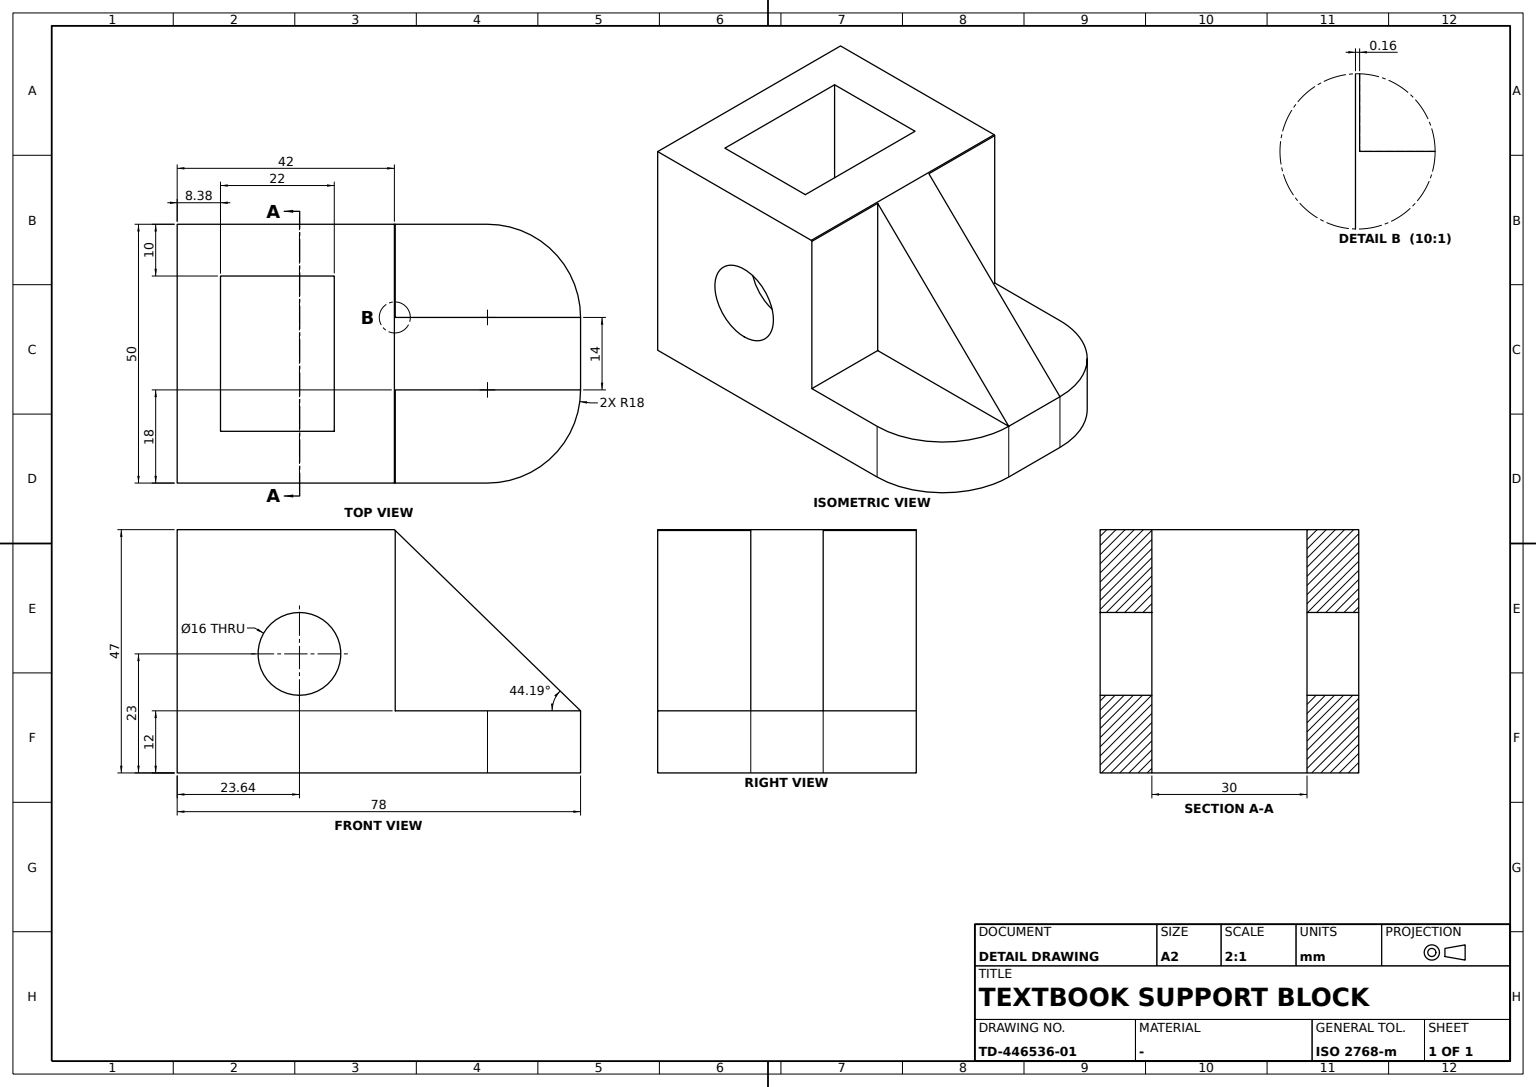
ISO-10303-21;
HEADER;
FILE_DESCRIPTION((''),'2;1');
FILE_NAME('','',(''),(''),'','','');
FILE_SCHEMA(('AUTOMOTIVE_DESIGN'));
ENDSEC;
DATA;
#1=APPLICATION_CONTEXT('');
#2=PRODUCT_CONTEXT('',#1,'mechanical');
#3=PRODUCT('','','',(#2));
#4=PRODUCT_DEFINITION_FORMATION('','',#3);
#5=PRODUCT_DEFINITION_CONTEXT('',#1,'design');
#6=PRODUCT_DEFINITION('','',#4,#5);
#7=PRODUCT_DEFINITION_SHAPE('','',#6);
#8=(LENGTH_UNIT()NAMED_UNIT(*)SI_UNIT(.MILLI.,.METRE.));
#9=(NAMED_UNIT(*)PLANE_ANGLE_UNIT()SI_UNIT($,.RADIAN.));
#10=(NAMED_UNIT(*)SI_UNIT($,.STERADIAN.)SOLID_ANGLE_UNIT());
#11=UNCERTAINTY_MEASURE_WITH_UNIT(LENGTH_MEASURE(0.005),#8,'distance_accuracy_value','');
#12=(GEOMETRIC_REPRESENTATION_CONTEXT(3)GLOBAL_UNCERTAINTY_ASSIGNED_CONTEXT((#11))GLOBAL_UNIT_ASSIGNED_CONTEXT((#8,#9,#10))REPRESENTATION_CONTEXT('',''));
#13=CARTESIAN_POINT('',(7.,42.160656,46.843807));
#14=VERTEX_POINT('',#13);
#15=CARTESIAN_POINT('',(7.,42.160656,12.));
#16=VERTEX_POINT('',#15);
#17=CARTESIAN_POINT('',(7.,42.160656,47.));
#18=DIRECTION('',(0.,0.,-1.));
#19=VECTOR('',#18,1000.);
#20=LINE('',#17,#19);
#21=EDGE_CURVE('',#14,#16,#20,.T.);
#22=ORIENTED_EDGE('',*,*,#21,.F.);
#23=CARTESIAN_POINT('',(25.,42.160656,46.843807));
#24=VERTEX_POINT('',#23);
#25=DIRECTION('',(-1.,0.,0.));
#26=VECTOR('',#25,1000.);
#27=LINE('',#23,#26);
#28=EDGE_CURVE('',#24,#14,#27,.T.);
#29=ORIENTED_EDGE('',*,*,#28,.F.);
#30=CARTESIAN_POINT('',(25.,42.160656,12.));
#31=VERTEX_POINT('',#30);
#32=CARTESIAN_POINT('',(25.,42.160656,47.));
#33=LINE('',#32,#19);
#34=EDGE_CURVE('',#24,#31,#33,.T.);
#35=ORIENTED_EDGE('',*,*,#34,.T.);
#36=LINE('',#30,#26);
#37=EDGE_CURVE('',#31,#16,#36,.T.);
#38=ORIENTED_EDGE('',*,*,#37,.T.);
#39=EDGE_LOOP('',(#22,#29,#35,#38));
#40=FACE_BOUND('',#39,.T.);
#41=DIRECTION('',(0.,1.,0.));
#42=AXIS2_PLACEMENT_3D('',#32,#41,#18);
#43=PLANE('',#42);
#44=ADVANCED_FACE('',(#40),#43,.T.);
#45=CARTESIAN_POINT('',(-25.,42.,47.));
#46=VERTEX_POINT('',#45);
#47=CARTESIAN_POINT('',(-25.,42.160656,46.843807));
#48=VERTEX_POINT('',#47);
#49=DIRECTION('',(0.,0.716994919,-0.697078393));
#50=VECTOR('',#49,1000.);
#51=LINE('',#45,#50);
#52=EDGE_CURVE('',#46,#48,#51,.T.);
#53=ORIENTED_EDGE('',*,*,#52,.T.);
#54=CARTESIAN_POINT('',(-25.,42.160656,12.));
#55=VERTEX_POINT('',#54);
#56=CARTESIAN_POINT('',(-25.,42.160656,47.));
#57=LINE('',#56,#19);
#58=EDGE_CURVE('',#48,#55,#57,.T.);
#59=ORIENTED_EDGE('',*,*,#58,.T.);
#60=CARTESIAN_POINT('',(-25.,60.,12.));
#61=VERTEX_POINT('',#60);
#62=VECTOR('',#41,1000.);
#63=LINE('',#54,#62);
#64=EDGE_CURVE('',#55,#61,#63,.T.);
#65=ORIENTED_EDGE('',*,*,#64,.T.);
#66=CARTESIAN_POINT('',(-25.,60.,0.));
#67=VERTEX_POINT('',#66);
#68=CARTESIAN_POINT('',(-25.,60.,23.5));
#69=LINE('',#68,#19);
#70=EDGE_CURVE('',#61,#67,#69,.T.);
#71=ORIENTED_EDGE('',*,*,#70,.T.);
#72=CARTESIAN_POINT('',(-25.,0.,0.));
#73=VERTEX_POINT('',#72);
#74=DIRECTION('',(0.,-1.,0.));
#75=VECTOR('',#74,1000.);
#76=LINE('',#72,#75);
#77=EDGE_CURVE('',#67,#73,#76,.T.);
#78=ORIENTED_EDGE('',*,*,#77,.T.);
#79=CARTESIAN_POINT('',(-25.,0.,47.));
#80=VERTEX_POINT('',#79);
#81=DIRECTION('',(0.,0.,1.));
#82=VECTOR('',#81,1000.);
#83=LINE('',#72,#82);
#84=EDGE_CURVE('',#73,#80,#83,.T.);
#85=ORIENTED_EDGE('',*,*,#84,.T.);
#86=LINE('',#79,#62);
#87=EDGE_CURVE('',#80,#46,#86,.T.);
#88=ORIENTED_EDGE('',*,*,#87,.T.);
#89=EDGE_LOOP('',(#53,#59,#65,#71,#78,#85,#88));
#90=FACE_BOUND('',#89,.T.);
#91=CARTESIAN_POINT('',(-25.,23.644327,15.));
#92=VERTEX_POINT('',#91);
#93=CARTESIAN_POINT('',(-25.,23.644327,23.));
#94=DIRECTION('',(1.,0.,0.));
#95=AXIS2_PLACEMENT_3D('',#93,#94,#18);
#96=CIRCLE('',#95,8.);
#97=EDGE_CURVE('',#92,#92,#96,.T.);
#98=ORIENTED_EDGE('',*,*,#97,.T.);
#99=EDGE_LOOP('',(#98));
#100=FACE_BOUND('',#99,.T.);
#101=AXIS2_PLACEMENT_3D('',#72,#94,#41);
#102=PLANE('',#101);
#103=ADVANCED_FACE('',(#90,#100),#102,.F.);
#104=CARTESIAN_POINT('',(25.,60.,12.));
#105=VERTEX_POINT('',#104);
#106=LINE('',#30,#62);
#107=EDGE_CURVE('',#31,#105,#106,.T.);
#108=ORIENTED_EDGE('',*,*,#107,.F.);
#109=ORIENTED_EDGE('',*,*,#34,.F.);
#110=CARTESIAN_POINT('',(25.,42.,47.));
#111=VERTEX_POINT('',#110);
#112=LINE('',#110,#50);
#113=EDGE_CURVE('',#111,#24,#112,.T.);
#114=ORIENTED_EDGE('',*,*,#113,.F.);
#115=CARTESIAN_POINT('',(25.,0.,47.));
#116=VERTEX_POINT('',#115);
#117=LINE('',#115,#62);
#118=EDGE_CURVE('',#116,#111,#117,.T.);
#119=ORIENTED_EDGE('',*,*,#118,.F.);
#120=CARTESIAN_POINT('',(25.,0.,0.));
#121=VERTEX_POINT('',#120);
#122=LINE('',#120,#82);
#123=EDGE_CURVE('',#121,#116,#122,.T.);
#124=ORIENTED_EDGE('',*,*,#123,.F.);
#125=CARTESIAN_POINT('',(25.,60.,0.));
#126=VERTEX_POINT('',#125);
#127=LINE('',#120,#75);
#128=EDGE_CURVE('',#126,#121,#127,.T.);
#129=ORIENTED_EDGE('',*,*,#128,.F.);
#130=CARTESIAN_POINT('',(25.,60.,23.5));
#131=LINE('',#130,#19);
#132=EDGE_CURVE('',#105,#126,#131,.T.);
#133=ORIENTED_EDGE('',*,*,#132,.F.);
#134=EDGE_LOOP('',(#108,#109,#114,#119,#124,#129,#133));
#135=FACE_BOUND('',#134,.T.);
#136=CARTESIAN_POINT('',(25.,23.644327,15.));
#137=VERTEX_POINT('',#136);
#138=CARTESIAN_POINT('',(25.,23.644327,23.));
#139=AXIS2_PLACEMENT_3D('',#138,#94,#18);
#140=CIRCLE('',#139,8.);
#141=EDGE_CURVE('',#137,#137,#140,.T.);
#142=ORIENTED_EDGE('',*,*,#141,.F.);
#143=EDGE_LOOP('',(#142));
#144=FACE_BOUND('',#143,.T.);
#145=AXIS2_PLACEMENT_3D('',#120,#94,#41);
#146=PLANE('',#145);
#147=ADVANCED_FACE('',(#135,#144),#146,.T.);
#148=CARTESIAN_POINT('',(-15.,8.375698,47.));
#149=VERTEX_POINT('',#148);
#150=CARTESIAN_POINT('',(-15.,8.375698,0.));
#151=VERTEX_POINT('',#150);
#152=LINE('',#148,#19);
#153=EDGE_CURVE('',#149,#151,#152,.T.);
#154=ORIENTED_EDGE('',*,*,#153,.T.);
#155=CARTESIAN_POINT('',(-15.,30.375698,0.));
#156=VERTEX_POINT('',#155);
#157=LINE('',#150,#62);
#158=EDGE_CURVE('',#151,#156,#157,.T.);
#159=ORIENTED_EDGE('',*,*,#158,.T.);
#160=CARTESIAN_POINT('',(-15.,30.375698,18.676963));
#161=VERTEX_POINT('',#160);
#162=CARTESIAN_POINT('',(-15.,30.375698,47.));
#163=LINE('',#162,#19);
#164=EDGE_CURVE('',#161,#156,#163,.T.);
#165=ORIENTED_EDGE('',*,*,#164,.F.);
#166=CARTESIAN_POINT('',(-15.,30.375698,27.323037));
#167=VERTEX_POINT('',#166);
#168=CARTESIAN_POINT('',(-15.,23.644327,23.));
#169=AXIS2_PLACEMENT_3D('',#168,#25,#81);
#170=CIRCLE('',#169,8.);
#171=EDGE_CURVE('',#161,#167,#170,.T.);
#172=ORIENTED_EDGE('',*,*,#171,.T.);
#173=VERTEX_POINT('',#162);
#174=EDGE_CURVE('',#173,#167,#163,.T.);
#175=ORIENTED_EDGE('',*,*,#174,.F.);
#176=CARTESIAN_POINT('',(-15.,0.,47.));
#177=LINE('',#176,#62);
#178=EDGE_CURVE('',#149,#173,#177,.T.);
#179=ORIENTED_EDGE('',*,*,#178,.F.);
#180=EDGE_LOOP('',(#154,#159,#165,#172,#175,#179));
#181=FACE_BOUND('',#180,.T.);
#182=AXIS2_PLACEMENT_3D('',#148,#25,#41);
#183=PLANE('',#182);
#184=ADVANCED_FACE('',(#181),#183,.F.);
#185=ORIENTED_EDGE('',*,*,#87,.F.);
#186=CARTESIAN_POINT('',(0.,0.,47.));
#187=VECTOR('',#94,1000.);
#188=LINE('',#186,#187);
#189=EDGE_CURVE('',#80,#116,#188,.T.);
#190=ORIENTED_EDGE('',*,*,#189,.T.);
#191=ORIENTED_EDGE('',*,*,#118,.T.);
#192=LINE('',#110,#26);
#193=EDGE_CURVE('',#111,#46,#192,.T.);
#194=ORIENTED_EDGE('',*,*,#193,.T.);
#195=EDGE_LOOP('',(#185,#190,#191,#194));
#196=FACE_BOUND('',#195,.T.);
#197=CARTESIAN_POINT('',(15.,30.375698,47.));
#198=VERTEX_POINT('',#197);
#199=CARTESIAN_POINT('',(15.,8.375698,47.));
#200=VERTEX_POINT('',#199);
#201=CARTESIAN_POINT('',(15.,0.,47.));
#202=LINE('',#201,#75);
#203=EDGE_CURVE('',#198,#200,#202,.T.);
#204=ORIENTED_EDGE('',*,*,#203,.T.);
#205=CARTESIAN_POINT('',(0.,8.375698,47.));
#206=LINE('',#205,#26);
#207=EDGE_CURVE('',#200,#149,#206,.T.);
#208=ORIENTED_EDGE('',*,*,#207,.T.);
#209=ORIENTED_EDGE('',*,*,#178,.T.);
#210=CARTESIAN_POINT('',(0.,30.375698,47.));
#211=LINE('',#210,#187);
#212=EDGE_CURVE('',#173,#198,#211,.T.);
#213=ORIENTED_EDGE('',*,*,#212,.T.);
#214=EDGE_LOOP('',(#204,#208,#209,#213));
#215=FACE_BOUND('',#214,.T.);
#216=AXIS2_PLACEMENT_3D('',#186,#18,#41);
#217=PLANE('',#216);
#218=ADVANCED_FACE('',(#196,#215),#217,.F.);
#219=CARTESIAN_POINT('',(-7.,78.,12.));
#220=VERTEX_POINT('',#219);
#221=CARTESIAN_POINT('',(-7.,42.160656,46.843807));
#222=VERTEX_POINT('',#221);
#223=CARTESIAN_POINT('',(-7.,43.899246,45.153511));
#224=DIRECTION('',(0.,-0.716994919,0.697078393));
#225=VECTOR('',#224,1000.);
#226=LINE('',#223,#225);
#227=EDGE_CURVE('',#220,#222,#226,.T.);
#228=ORIENTED_EDGE('',*,*,#227,.F.);
#229=CARTESIAN_POINT('',(-7.,42.160656,12.));
#230=VERTEX_POINT('',#229);
#231=LINE('',#229,#62);
#232=EDGE_CURVE('',#230,#220,#231,.T.);
#233=ORIENTED_EDGE('',*,*,#232,.F.);
#234=CARTESIAN_POINT('',(-7.,42.160656,47.));
#235=LINE('',#234,#19);
#236=EDGE_CURVE('',#222,#230,#235,.T.);
#237=ORIENTED_EDGE('',*,*,#236,.F.);
#238=EDGE_LOOP('',(#228,#233,#237));
#239=FACE_BOUND('',#238,.T.);
#240=CARTESIAN_POINT('',(-7.,0.,0.));
#241=AXIS2_PLACEMENT_3D('',#240,#94,#41);
#242=PLANE('',#241);
#243=ADVANCED_FACE('',(#239),#242,.F.);
#244=CARTESIAN_POINT('',(15.,8.375698,0.));
#245=VERTEX_POINT('',#244);
#246=LINE('',#199,#19);
#247=EDGE_CURVE('',#200,#245,#246,.T.);
#248=ORIENTED_EDGE('',*,*,#247,.T.);
#249=LINE('',#244,#26);
#250=EDGE_CURVE('',#245,#151,#249,.T.);
#251=ORIENTED_EDGE('',*,*,#250,.T.);
#252=ORIENTED_EDGE('',*,*,#153,.F.);
#253=ORIENTED_EDGE('',*,*,#207,.F.);
#254=EDGE_LOOP('',(#248,#251,#252,#253));
#255=FACE_BOUND('',#254,.T.);
#256=AXIS2_PLACEMENT_3D('',#199,#74,#25);
#257=PLANE('',#256);
#258=ADVANCED_FACE('',(#255),#257,.F.);
#259=CARTESIAN_POINT('',(-7.,78.,0.));
#260=VERTEX_POINT('',#259);
#261=CARTESIAN_POINT('',(-7.,78.,23.5));
#262=LINE('',#261,#19);
#263=EDGE_CURVE('',#220,#260,#262,.T.);
#264=ORIENTED_EDGE('',*,*,#263,.F.);
#265=CARTESIAN_POINT('',(7.,78.,12.));
#266=VERTEX_POINT('',#265);
#267=CARTESIAN_POINT('',(0.,78.,12.));
#268=LINE('',#267,#26);
#269=EDGE_CURVE('',#266,#220,#268,.T.);
#270=ORIENTED_EDGE('',*,*,#269,.F.);
#271=CARTESIAN_POINT('',(7.,78.,0.));
#272=VERTEX_POINT('',#271);
#273=CARTESIAN_POINT('',(7.,78.,23.5));
#274=LINE('',#273,#19);
#275=EDGE_CURVE('',#266,#272,#274,.T.);
#276=ORIENTED_EDGE('',*,*,#275,.T.);
#277=CARTESIAN_POINT('',(0.,78.,0.));
#278=LINE('',#277,#187);
#279=EDGE_CURVE('',#260,#272,#278,.T.);
#280=ORIENTED_EDGE('',*,*,#279,.F.);
#281=EDGE_LOOP('',(#264,#270,#276,#280));
#282=FACE_BOUND('',#281,.T.);
#283=CARTESIAN_POINT('',(0.,78.,47.));
#284=AXIS2_PLACEMENT_3D('',#283,#74,#18);
#285=PLANE('',#284);
#286=ADVANCED_FACE('',(#282),#285,.F.);
#287=ORIENTED_EDGE('',*,*,#37,.F.);
#288=ORIENTED_EDGE('',*,*,#107,.T.);
#289=CARTESIAN_POINT('',(7.,60.,12.));
#290=AXIS2_PLACEMENT_3D('',#289,#81,#94);
#291=CIRCLE('',#290,18.);
#292=EDGE_CURVE('',#105,#266,#291,.T.);
#293=ORIENTED_EDGE('',*,*,#292,.T.);
#294=LINE('',#15,#62);
#295=EDGE_CURVE('',#16,#266,#294,.T.);
#296=ORIENTED_EDGE('',*,*,#295,.F.);
#297=EDGE_LOOP('',(#287,#288,#293,#296));
#298=FACE_BOUND('',#297,.T.);
#299=AXIS2_PLACEMENT_3D('',#30,#81,#41);
#300=PLANE('',#299);
#301=ADVANCED_FACE('',(#298),#300,.T.);
#302=ORIENTED_EDGE('',*,*,#97,.F.);
#303=EDGE_LOOP('',(#302));
#304=FACE_BOUND('',#303,.T.);
#305=ORIENTED_EDGE('',*,*,#141,.T.);
#306=EDGE_LOOP('',(#305));
#307=FACE_BOUND('',#306,.T.);
#308=ORIENTED_EDGE('',*,*,#171,.F.);
#309=CARTESIAN_POINT('',(15.,30.375698,18.676963));
#310=VERTEX_POINT('',#309);
#311=LINE('',#160,#187);
#312=EDGE_CURVE('',#161,#310,#311,.T.);
#313=ORIENTED_EDGE('',*,*,#312,.T.);
#314=CARTESIAN_POINT('',(15.,30.375698,27.323037));
#315=VERTEX_POINT('',#314);
#316=CARTESIAN_POINT('',(15.,23.644327,23.));
#317=AXIS2_PLACEMENT_3D('',#316,#94,#18);
#318=CIRCLE('',#317,8.);
#319=EDGE_CURVE('',#315,#310,#318,.T.);
#320=ORIENTED_EDGE('',*,*,#319,.F.);
#321=LINE('',#166,#187);
#322=EDGE_CURVE('',#315,#167,#321,.F.);
#323=ORIENTED_EDGE('',*,*,#322,.T.);
#324=EDGE_LOOP('',(#308,#313,#320,#323));
#325=FACE_BOUND('',#324,.T.);
#326=CARTESIAN_POINT('',(-24.9,23.644327,23.));
#327=AXIS2_PLACEMENT_3D('',#326,#94,#41);
#328=CYLINDRICAL_SURFACE('',#327,8.);
#329=ADVANCED_FACE('',(#304,#307,#325),#328,.F.);
#330=ORIENTED_EDGE('',*,*,#275,.F.);
#331=ORIENTED_EDGE('',*,*,#292,.F.);
#332=ORIENTED_EDGE('',*,*,#132,.T.);
#333=CARTESIAN_POINT('',(7.,60.,0.));
#334=AXIS2_PLACEMENT_3D('',#333,#81,#94);
#335=CIRCLE('',#334,18.);
#336=EDGE_CURVE('',#126,#272,#335,.T.);
#337=ORIENTED_EDGE('',*,*,#336,.T.);
#338=EDGE_LOOP('',(#330,#331,#332,#337));
#339=FACE_BOUND('',#338,.T.);
#340=CARTESIAN_POINT('',(7.,60.,23.5));
#341=AXIS2_PLACEMENT_3D('',#340,#18,#41);
#342=CYLINDRICAL_SURFACE('',#341,18.);
#343=ADVANCED_FACE('',(#339),#342,.T.);
#344=ORIENTED_EDGE('',*,*,#64,.F.);
#345=LINE('',#30,#187);
#346=EDGE_CURVE('',#55,#230,#345,.T.);
#347=ORIENTED_EDGE('',*,*,#346,.T.);
#348=ORIENTED_EDGE('',*,*,#232,.T.);
#349=CARTESIAN_POINT('',(-7.,60.,12.));
#350=AXIS2_PLACEMENT_3D('',#349,#81,#94);
#351=CIRCLE('',#350,18.);
#352=EDGE_CURVE('',#220,#61,#351,.T.);
#353=ORIENTED_EDGE('',*,*,#352,.T.);
#354=EDGE_LOOP('',(#344,#347,#348,#353));
#355=FACE_BOUND('',#354,.T.);
#356=ADVANCED_FACE('',(#355),#300,.T.);
#357=LINE('',#23,#187);
#358=EDGE_CURVE('',#48,#222,#357,.T.);
#359=ORIENTED_EDGE('',*,*,#358,.T.);
#360=ORIENTED_EDGE('',*,*,#236,.T.);
#361=ORIENTED_EDGE('',*,*,#346,.F.);
#362=ORIENTED_EDGE('',*,*,#58,.F.);
#363=EDGE_LOOP('',(#359,#360,#361,#362));
#364=FACE_BOUND('',#363,.T.);
#365=ADVANCED_FACE('',(#364),#43,.T.);
#366=ORIENTED_EDGE('',*,*,#123,.T.);
#367=ORIENTED_EDGE('',*,*,#189,.F.);
#368=ORIENTED_EDGE('',*,*,#84,.F.);
#369=CARTESIAN_POINT('',(0.,0.,0.));
#370=LINE('',#369,#187);
#371=EDGE_CURVE('',#73,#121,#370,.T.);
#372=ORIENTED_EDGE('',*,*,#371,.T.);
#373=EDGE_LOOP('',(#366,#367,#368,#372));
#374=FACE_BOUND('',#373,.T.);
#375=AXIS2_PLACEMENT_3D('',#369,#41,#81);
#376=PLANE('',#375);
#377=ADVANCED_FACE('',(#374),#376,.F.);
#378=ORIENTED_EDGE('',*,*,#352,.F.);
#379=ORIENTED_EDGE('',*,*,#263,.T.);
#380=CARTESIAN_POINT('',(-7.,60.,0.));
#381=AXIS2_PLACEMENT_3D('',#380,#81,#94);
#382=CIRCLE('',#381,18.);
#383=EDGE_CURVE('',#260,#67,#382,.T.);
#384=ORIENTED_EDGE('',*,*,#383,.T.);
#385=ORIENTED_EDGE('',*,*,#70,.F.);
#386=EDGE_LOOP('',(#378,#379,#384,#385));
#387=FACE_BOUND('',#386,.T.);
#388=CARTESIAN_POINT('',(-7.,60.,23.5));
#389=AXIS2_PLACEMENT_3D('',#388,#18,#25);
#390=CYLINDRICAL_SURFACE('',#389,18.);
#391=ADVANCED_FACE('',(#387),#390,.T.);
#392=ORIENTED_EDGE('',*,*,#322,.F.);
#393=LINE('',#197,#19);
#394=EDGE_CURVE('',#198,#315,#393,.T.);
#395=ORIENTED_EDGE('',*,*,#394,.F.);
#396=ORIENTED_EDGE('',*,*,#212,.F.);
#397=ORIENTED_EDGE('',*,*,#174,.T.);
#398=EDGE_LOOP('',(#392,#395,#396,#397));
#399=FACE_BOUND('',#398,.T.);
#400=AXIS2_PLACEMENT_3D('',#162,#41,#94);
#401=PLANE('',#400);
#402=ADVANCED_FACE('',(#399),#401,.F.);
#403=ORIENTED_EDGE('',*,*,#295,.T.);
#404=CARTESIAN_POINT('',(7.,43.899246,45.153511));
#405=LINE('',#404,#225);
#406=EDGE_CURVE('',#266,#14,#405,.T.);
#407=ORIENTED_EDGE('',*,*,#406,.T.);
#408=ORIENTED_EDGE('',*,*,#21,.T.);
#409=EDGE_LOOP('',(#403,#407,#408));
#410=FACE_BOUND('',#409,.T.);
#411=CARTESIAN_POINT('',(7.,0.,0.));
#412=AXIS2_PLACEMENT_3D('',#411,#94,#41);
#413=PLANE('',#412);
#414=ADVANCED_FACE('',(#410),#413,.T.);
#415=ORIENTED_EDGE('',*,*,#113,.T.);
#416=ORIENTED_EDGE('',*,*,#28,.T.);
#417=ORIENTED_EDGE('',*,*,#406,.F.);
#418=ORIENTED_EDGE('',*,*,#269,.T.);
#419=ORIENTED_EDGE('',*,*,#227,.T.);
#420=ORIENTED_EDGE('',*,*,#358,.F.);
#421=ORIENTED_EDGE('',*,*,#52,.F.);
#422=ORIENTED_EDGE('',*,*,#193,.F.);
#423=EDGE_LOOP('',(#415,#416,#417,#418,#419,#420,#421,#422));
#424=FACE_BOUND('',#423,.T.);
#425=DIRECTION('',(0.,0.697078393,0.716994919));
#426=AXIS2_PLACEMENT_3D('',#110,#425,#49);
#427=PLANE('',#426);
#428=ADVANCED_FACE('',(#424),#427,.T.);
#429=ORIENTED_EDGE('',*,*,#247,.F.);
#430=ORIENTED_EDGE('',*,*,#203,.F.);
#431=ORIENTED_EDGE('',*,*,#394,.T.);
#432=ORIENTED_EDGE('',*,*,#319,.T.);
#433=CARTESIAN_POINT('',(15.,30.375698,0.));
#434=VERTEX_POINT('',#433);
#435=EDGE_CURVE('',#310,#434,#393,.T.);
#436=ORIENTED_EDGE('',*,*,#435,.T.);
#437=LINE('',#433,#75);
#438=EDGE_CURVE('',#434,#245,#437,.T.);
#439=ORIENTED_EDGE('',*,*,#438,.T.);
#440=EDGE_LOOP('',(#429,#430,#431,#432,#436,#439));
#441=FACE_BOUND('',#440,.T.);
#442=AXIS2_PLACEMENT_3D('',#197,#94,#74);
#443=PLANE('',#442);
#444=ADVANCED_FACE('',(#441),#443,.F.);
#445=LINE('',#155,#187);
#446=EDGE_CURVE('',#156,#434,#445,.T.);
#447=ORIENTED_EDGE('',*,*,#446,.F.);
#448=ORIENTED_EDGE('',*,*,#158,.F.);
#449=ORIENTED_EDGE('',*,*,#250,.F.);
#450=ORIENTED_EDGE('',*,*,#438,.F.);
#451=EDGE_LOOP('',(#447,#448,#449,#450));
#452=FACE_BOUND('',#451,.T.);
#453=ORIENTED_EDGE('',*,*,#336,.F.);
#454=ORIENTED_EDGE('',*,*,#128,.T.);
#455=ORIENTED_EDGE('',*,*,#371,.F.);
#456=ORIENTED_EDGE('',*,*,#77,.F.);
#457=ORIENTED_EDGE('',*,*,#383,.F.);
#458=ORIENTED_EDGE('',*,*,#279,.T.);
#459=EDGE_LOOP('',(#453,#454,#455,#456,#457,#458));
#460=FACE_BOUND('',#459,.T.);
#461=AXIS2_PLACEMENT_3D('',#277,#81,#74);
#462=PLANE('',#461);
#463=ADVANCED_FACE('',(#452,#460),#462,.F.);
#464=ORIENTED_EDGE('',*,*,#446,.T.);
#465=ORIENTED_EDGE('',*,*,#435,.F.);
#466=ORIENTED_EDGE('',*,*,#312,.F.);
#467=ORIENTED_EDGE('',*,*,#164,.T.);
#468=EDGE_LOOP('',(#464,#465,#466,#467));
#469=FACE_BOUND('',#468,.T.);
#470=ADVANCED_FACE('',(#469),#401,.F.);
#471=CLOSED_SHELL('',(#44,#103,#147,#184,#218,#243,#258,#286,#301,#329,#343,#356,#365,#377,#391,#402,#414,#428,#444,#463,#470));
#472=MANIFOLD_SOLID_BREP('',#471);
#473=ADVANCED_BREP_SHAPE_REPRESENTATION('',(#472),#12);
#474=SHAPE_DEFINITION_REPRESENTATION(#7,#473);
ENDSEC;
END-ISO-10303-21;
